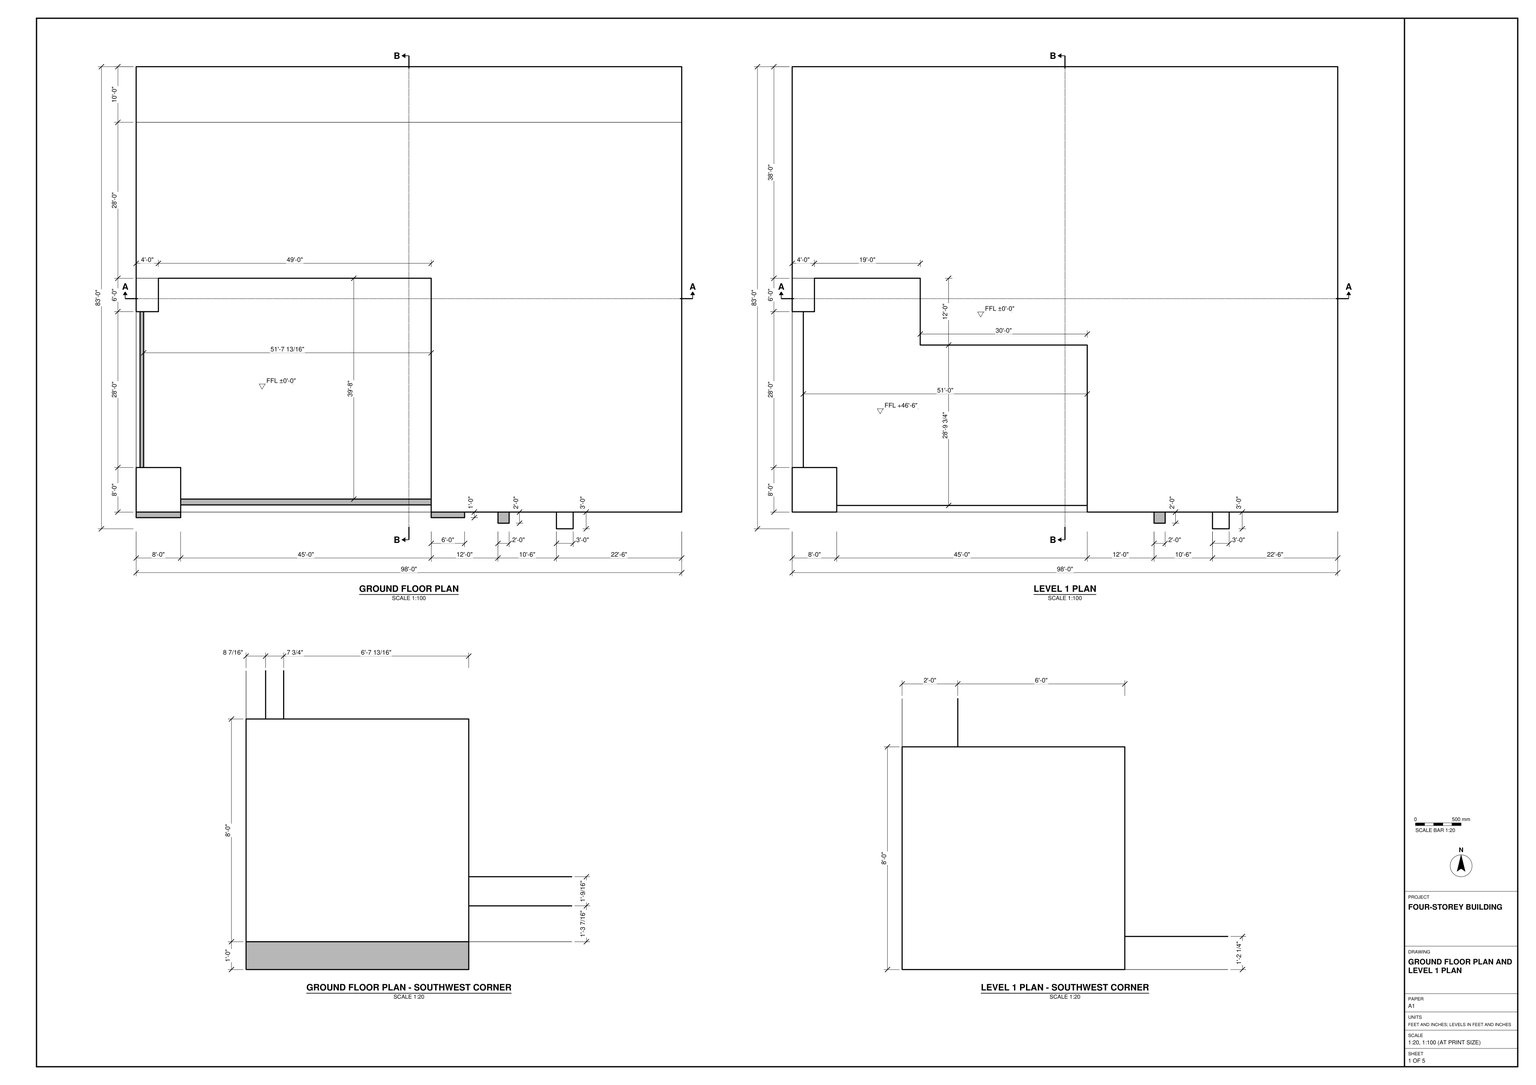
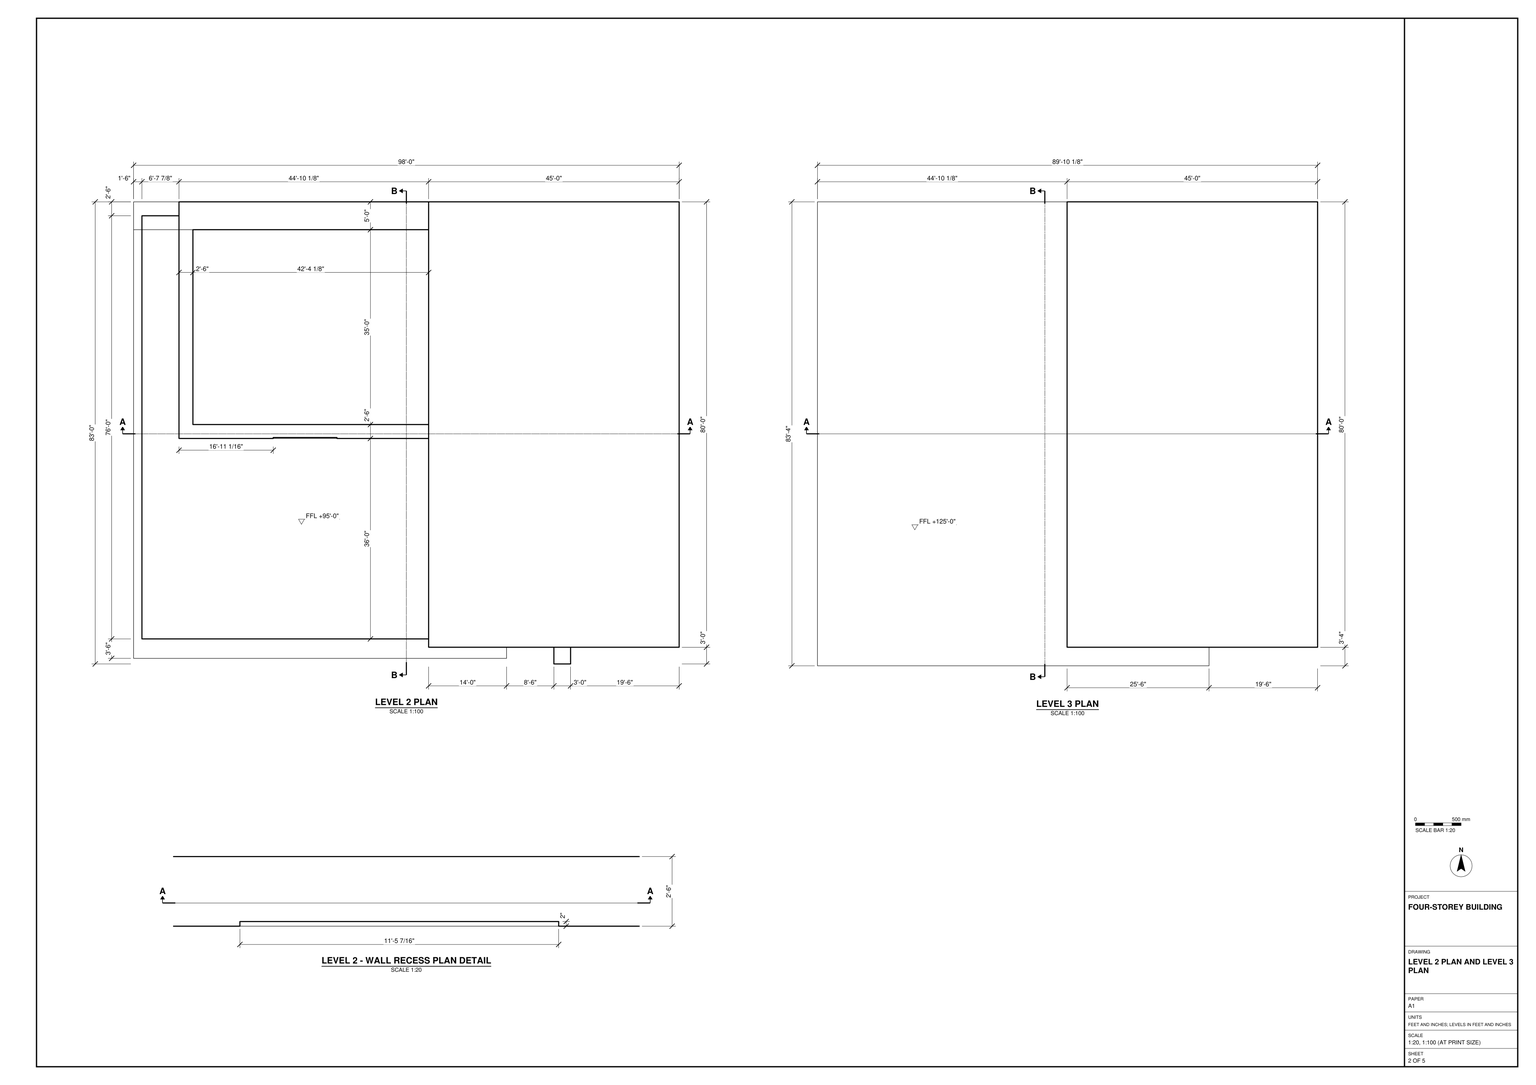
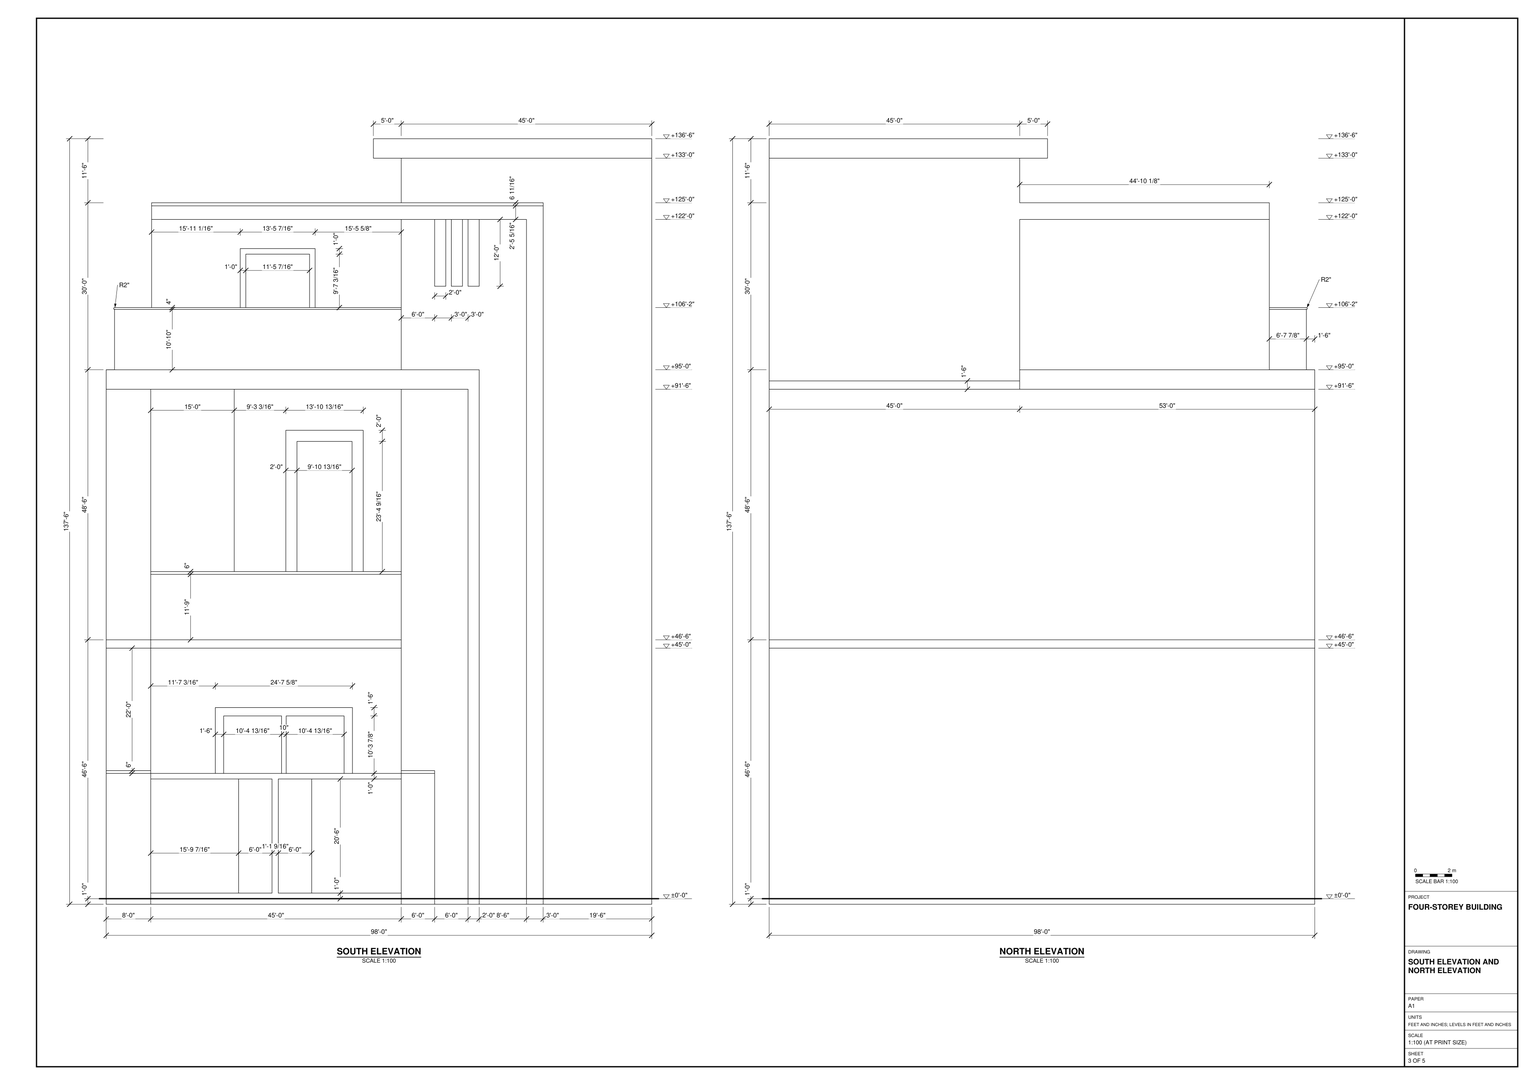
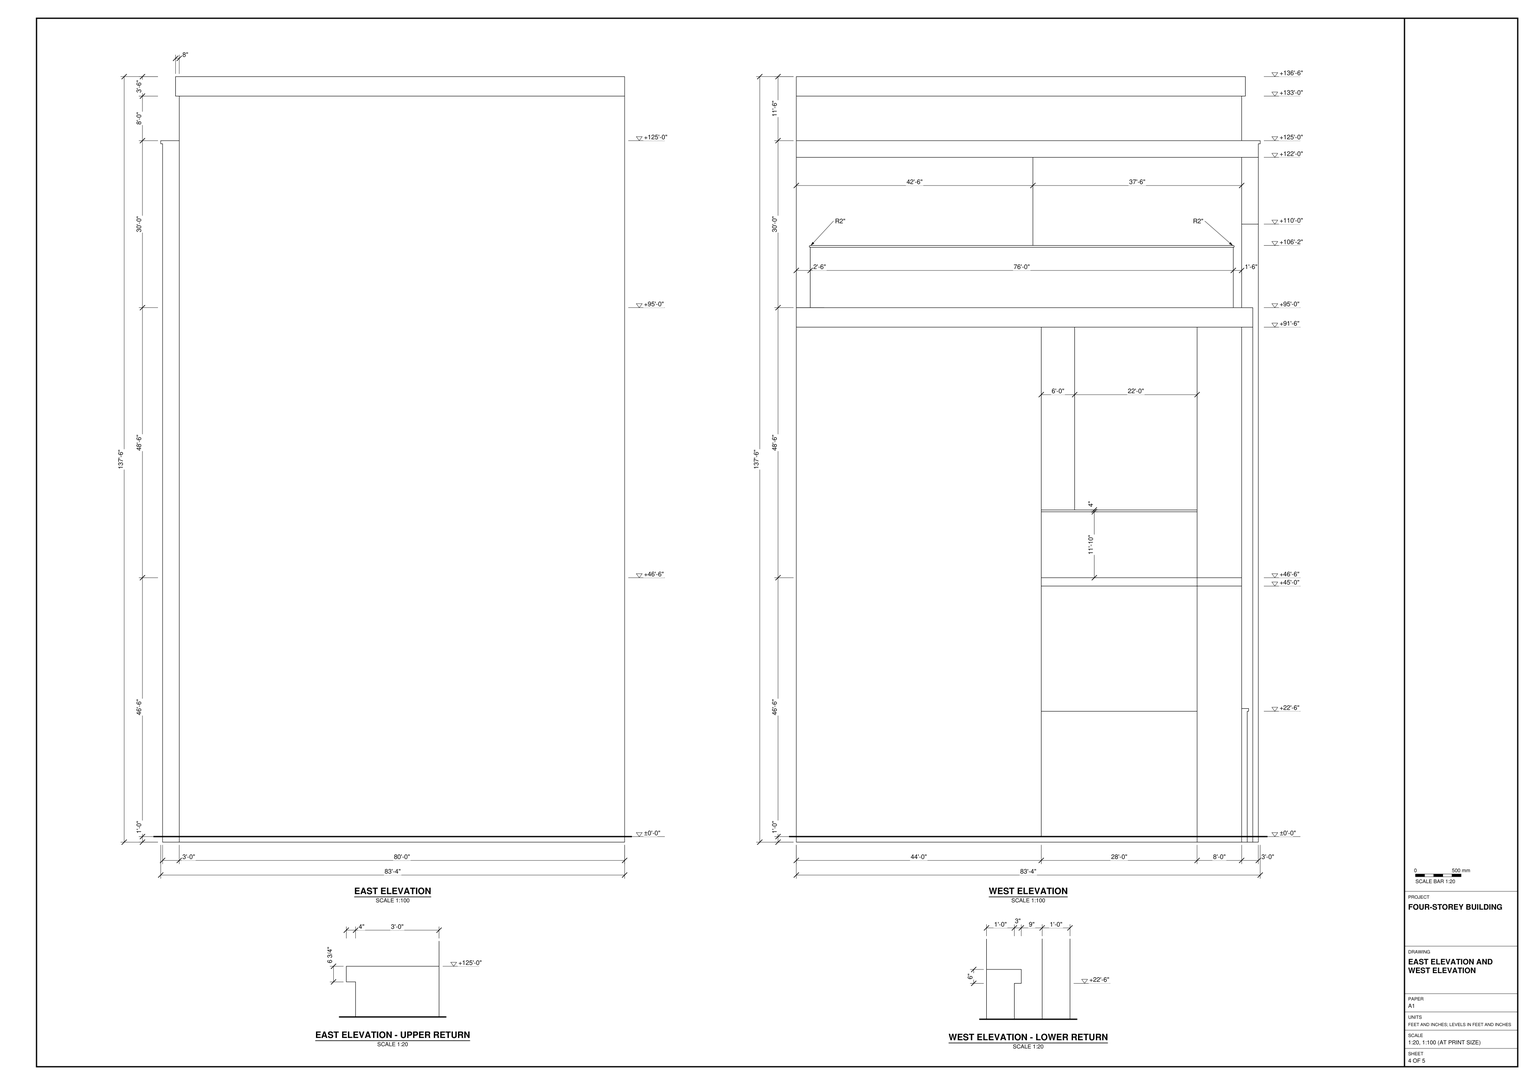
Build the four-storey building in SketchUp from task_files/diagram_01.pdf. Work in feet and inches. The overall dimensions are 98'-0" east to west, 83'-4" north to south and 137'-6" from the underside of the base to the top of the roof. Set the ground floor at ±0'-0" and the successive floor levels at +46'-6", +95'-0" and +125'-0".

Use the floor plans to locate the walls, slab edges and supports. Follow the enlarged southwest corner details: the adjoining edges meet the corner pier at different offsets on the ground floor and Level 1. Form the stepped bay on Level 1 and the shallow wall recess on Level 2. Use the wall and slab thicknesses shown rather than giving all elements a common thickness.

Match the south elevation’s framed openings, horizontal bands and vertical returns. Keep the highest volume on the east side and extend its flat roof cap westward as drawn. Group walls, slabs and roofs separately. Keep each furniture or joinery piece shown in its own group or component, and use components for repeated parts. Decor and loose items may be any suitable library components. Save one SketchUp model as output_files/four_storey_building_with_stepped_facades.skp.

# SketchUp Ruby script. Lengths in inches.
U = 1.inch
M = Sketchup.active_model
def pt(a) = Geom::Point3d.new(a.map { |v| v * U })
def face(e, loops, mat)
  f = e.add_face(loops[0].map { |a| pt(a) })
  loops[1..].each { |l| e.add_face(l.map { |a| pt(a) }).erase! }
  f.material = f.back_material = mat if mat
  f
end
# faces: each face lists its corners as indices into pts; further lists are holes
def faces(e, pts, list, mat = nil) = list.each { |f| face(e, (f[0].is_a?(Array) ? f : [f]).map { |l| l.map { |i| pts[i] } }, mat) }
# xy, xz, yz: faces in a plane at the given z, y or x. An outline is a flat list of corners, or four numbers for a rectangle; further outlines are holes
def ring(l) = l.size == 4 ? [[l[0], l[1]], [l[2], l[1]], [l[2], l[3]], [l[0], l[3]]] : l.each_slice(2).to_a
def flat(e, list, mat, &to3) = list.each { |f| face(e, (f[0].is_a?(Array) ? f : [f]).map { |l| ring(l).map { |u, v| to3.(u, v) } }, mat) }
def xy(e, z, list, mat = nil) = flat(e, list, mat) { |x, y| [x, y, z] }
def xz(e, y, list, mat = nil) = flat(e, list, mat) { |x, z| [x, y, z] }
def yz(e, x, list, mat = nil) = flat(e, list, mat) { |y, z| [x, y, z] }
def lines(e, pts, list) = list.each { |a, b| e.add_line(pt(pts[a]), pt(pts[b])) }
# prism: a flat outline (further loops are holes) pulled along v
def prism(e, loops, v, mat = nil)
  f = face(e, loops, mat); d = Geom::Vector3d.new(v.map { |x| x * U })
  f.pushpull(f.normal.samedirection?(d) ? d.length : -d.length)
end
def box(e, o, s, mat = nil) = prism(e, [[o, [o[0] + s[0], o[1], o[2]], [o[0] + s[0], o[1] + s[1], o[2]], [o[0], o[1] + s[1], o[2]]]], [0, 0, s[2]], mat)
def at(x, y, z, deg = 0) = Geom::Transformation.translation(pt([x, y, z])) * Geom::Transformation.rotation(ORIGIN, Z_AXIS, deg.degrees)
def axes(o, x, y, z) = Geom::Transformation.new([*x, 0, *y, 0, *z, 0, *pt(o).to_a, 1])
def part(name) = M.definitions.add(name)
# library, detail: a bought-in or finely detailed component or shape, given as its bounding box
def library(name, o, s) = part(name).tap { |d| box(d.entities, o, s) }
def detail(e, o, s) = box(e.add_group.entities, o, s)
def put(e, d, t, mat = nil) = e.add_instance(d, t).tap { |i| i.material = mat if mat }
def group(e, t, mat = nil) = e.add_group.tap { |g| g.transformation = t; g.material = mat if mat }.entities
root = M.entities
M.materials.add("[0009_Linen]").color = [250, 240, 230]
M.materials.add("[0051_Cornsilk]").color = [255, 248, 220]
M.materials.add("[0061_OliveDrab]").color = [53, 71, 17]
M.materials.add("[0061_OliveDrab]1").color = [71, 94, 23]
M.materials.add("[0118_Thistle]").color = [216, 191, 216]
M.materials.add("[0132_LightGray]").color = [169, 169, 169]
M.materials.add("[0135_DarkGray]").color = [81, 81, 81]
M.materials.add("[0136_Charcoal]").color = [17, 17, 17]
M.materials.add("[Carrera Marble]").color = [165, 165, 165]
M.materials.add("[Checker Plate]").color = [247, 247, 247]
M.materials.add("[Cladding Siding Tan]").color = [90, 119, 67]
M.materials.add("[Cladding Siding Tan]1").color = [127, 71, 26]
M.materials.add("[Stone Marble]").color = [143, 138, 136]
M.materials.add("[Translucent Glass Gray]").color = [128, 128, 128]
M.materials["[Translucent Glass Gray]"].alpha = 0.5
xy(root,0,[[906,4,942,40],[780,16,804,40],[0,28,96,40],[636,28,708,40],[0,40,1176,880],
  [0,880,1176,1000]])
xy(root,12,[[96,55.44,636,68.01],[8.43,136,16.2,472],[0,472,48,544]])
xy(root,12,[[96,40,636,55.44],[96,68.01,636,68.01,636,544,48,544,48,472,16.2,472,16.2,136,96,136],[0,136,8.43,472]],"[Stone Marble]")
xy(root,126.9,[[253.2,544,378.01,546],[388.01,544,512.83,546]])
xy(root,282,[[0,25,96,28],[636,25,708,28]])
xy(root,282,[[96,55.44,636,68.01],[8.43,136,16.2,472]],"[0009_Linen]")
xy(root,288,[[0,25,96,40],[636,25,708,40]],"[0061_OliveDrab]")
xy(root,405.9,[[253.2,544,378.01,546],[388.01,544,512.83,546]])
xy(root,552,[[220.83,139.21,217.72,139.57,214.81,140.72,212.29,142.58,210.34,145.03,209.09,147.9,208.63,151,208.98,154.12,210.13,157.03,212,159.55,214.45,161.5,217.32,162.75,220.42,163.21,223.53,162.85,226.45,161.7,228.96,159.84,230.91,157.39,232.16,154.52,232.625,151.42,232.27,148.3,231.12,145.39,229.26,142.87,226.8,140.92,223.93,139.67],[444.46,139.21,441.35,139.57,438.43,140.72,435.91,142.58,433.96,145.03,432.72,147.9,432.25,151,432.61,154.12,433.76,157.03,435.62,159.55,438.07,161.5,440.95,162.75,444.04,163.21,447.16,162.85,450.07,161.7,452.59,159.84,454.54,157.39,455.79,154.52,456.25,151.42,455.89,148.3,454.75,145.39,452.88,142.87,450.43,140.92,447.56,139.67],[198.83,349.52,195.72,349.88,192.81,351.03,190.29,352.89,188.34,355.34,187.09,358.22,186.63,361.32,186.98,364.43,188.13,367.34,190,369.86,192.45,371.81,195.32,373.06,198.42,373.52,201.53,373.17,204.45,372.02,206.96,370.15,208.91,367.7,210.16,364.83,210.625,361.73,210.27,358.62,209.12,355.7,207.26,353.18,204.8,351.24,201.93,349.99],[444.46,349.52,441.35,349.88,438.43,351.03,435.91,352.89,433.96,355.34,432.72,358.22,432.25,361.32,432.61,364.43,433.76,367.34,435.62,369.86,438.07,371.81,440.95,373.06,444.04,373.52,447.16,373.17,450.07,372.02,452.59,370.15,454.54,367.7,455.79,364.83,456.25,361.73,455.89,358.62,454.75,355.7,452.88,353.18,450.43,351.24,447.56,349.99]])
xy(root,552,[[[96,40,96,136,0,136,0,472,48,472,48,544,636,544,636,40],[220.83,139.21,223.93,139.67,226.8,140.92,229.26,142.87,231.12,145.39,232.27,148.3,232.625,151.42,232.16,154.52,230.91,157.39,228.96,159.84,226.45,161.7,223.53,162.85,220.42,163.21,217.32,162.75,214.45,161.5,212,159.55,210.13,157.03,208.98,154.12,208.63,151,209.09,147.9,210.34,145.03,212.29,142.58,214.81,140.72,217.72,139.57],[444.46,139.21,447.56,139.67,450.43,140.92,452.88,142.87,454.75,145.39,455.89,148.3,456.25,151.42,455.79,154.52,454.54,157.39,452.59,159.84,450.07,161.7,447.16,162.85,444.04,163.21,440.95,162.75,438.07,161.5,435.62,159.55,433.76,157.03,432.61,154.12,432.25,151,432.72,147.9,433.96,145.03,435.91,142.58,438.43,140.72,441.35,139.57],[444.46,349.52,447.56,349.99,450.43,351.24,452.88,353.18,454.75,355.7,455.89,358.62,456.25,361.73,455.79,364.83,454.54,367.7,452.59,370.15,450.07,372.02,447.16,373.17,444.04,373.52,440.95,373.06,438.07,371.81,435.62,369.86,433.76,367.34,432.61,364.43,432.25,361.32,432.72,358.22,433.96,355.34,435.91,352.89,438.43,351.03,441.35,349.88],[198.83,349.52,201.93,349.99,204.8,351.24,207.26,353.18,209.12,355.7,210.27,358.62,210.625,361.73,210.16,364.83,208.91,367.7,206.96,370.15,204.45,372.02,201.53,373.17,198.42,373.52,195.32,373.06,192.45,371.81,190,369.86,188.13,367.34,186.98,364.43,186.63,361.32,187.09,358.22,188.34,355.34,190.29,352.89,192.81,351.03,195.72,349.88]]],"[0118_Thistle]")
xy(root,570,[[0,40,96,136]])
xy(root,570,[[96,40,636,54.26],[0,136,24,472]],"[0051_Cornsilk]")
xy(root,570,[[96,54.26,636,54.26,636,400,276,400,276,544,48,544,48,472,24,472,24,136,96,136]],"[Carrera Marble]")
xy(root,657.21,[[411.19,400,530.01,402]])
xy(root,997.58,[[411.19,400,530.01,402]])
xy(root,1110,[[0,16,96,40],[215.45,103.5,212.32,103.56,209.31,104.42,206.62,106.03,204.44,108.28,202.92,111.02,202.16,114.0625,202.22,117.19,203.08,120.2,204.69,122.89,206.94,125.07,209.68,126.59,212.72,127.35,215.85,127.3,218.86,126.43,221.55,124.82,223.73,122.57,225.25,119.83,226.01,116.79,225.96,113.66,225.09,110.65,223.48,107.96,221.23,105.78,218.49,104.26],[467.01,103.5,463.88,103.56,460.87,104.42,458.18,106.03,456.01,108.28,454.49,111.02,453.73,114.0625,453.78,117.19,454.64,120.2,456.25,122.89,458.51,125.07,461.24,126.59,464.28,127.35,467.42,127.3,470.43,126.43,473.11,124.82,475.29,122.57,476.8125,119.83,477.57,116.79,477.52,113.66,476.66,110.65,475.04,107.96,472.79,105.78,470.05,104.26],[197.51,304.07,194.38,304.12,191.37,304.98,188.68,306.59,186.51,308.85,184.99,311.58,184.23,314.625,184.28,317.76,185.14,320.77,186.75,323.45,189.01,325.63,191.74,327.15,194.78,327.91,197.92,327.86,200.93,327,203.61,325.38,205.79,323.13,207.3125,320.39,208.07,317.35,208.02,314.22,207.16,311.21,205.54,308.52,203.29,306.35,200.55,304.83],[467.01,304.07,463.88,304.12,460.87,304.98,458.18,306.59,456.01,308.85,454.49,311.58,453.73,314.625,453.78,317.76,454.64,320.77,456.25,323.45,458.51,325.63,461.24,327.15,464.28,327.91,467.42,327.86,470.43,327,473.11,325.38,475.29,323.13,476.8125,320.39,477.57,317.35,477.52,314.22,476.66,311.21,475.04,308.52,472.79,306.35,470.05,304.83],
  [0,472,48,544]])
xy(root,1110,[[[96,16,96,136,0,136,0,472,48,472,48,544,276,544,276,400,636,400,636,40,780,40,780,16],[215.45,103.5,218.49,104.26,221.23,105.78,223.48,107.96,225.09,110.65,225.96,113.66,226.01,116.79,225.25,119.83,223.73,122.57,221.55,124.82,218.86,126.43,215.85,127.3,212.72,127.35,209.68,126.59,206.94,125.07,204.69,122.89,203.08,120.2,202.22,117.19,202.16,114.0625,202.92,111.02,204.44,108.28,206.62,106.03,209.31,104.42,212.32,103.56],[467.01,103.5,470.05,104.26,472.79,105.78,475.04,107.96,476.66,110.65,477.52,113.66,477.57,116.79,476.8125,119.83,475.29,122.57,473.11,124.82,470.43,126.43,467.42,127.3,464.28,127.35,461.24,126.59,458.51,125.07,456.25,122.89,454.64,120.2,453.78,117.19,453.73,114.0625,454.49,111.02,456.01,108.28,458.18,106.03,460.87,104.42,463.88,103.56],[467.01,304.07,470.05,304.83,472.79,306.35,475.04,308.52,476.66,311.21,477.52,314.22,477.57,317.35,476.8125,320.39,475.29,323.13,473.11,325.38,470.43,327,467.42,327.86,464.28,327.91,461.24,327.15,458.51,325.63,456.25,323.45,454.64,320.77,453.78,317.76,453.73,314.625,454.49,311.58,456.01,308.85,458.18,306.59,460.87,304.98,463.88,304.12],[197.51,304.07,200.55,304.83,203.29,306.35,205.54,308.52,207.16,311.21,208.02,314.22,208.07,317.35,207.3125,320.39,205.79,323.13,203.61,325.38,200.93,327,197.92,327.86,194.78,327.91,191.74,327.15,189.01,325.63,186.75,323.45,185.14,320.77,184.28,317.76,184.23,314.625,184.99,311.58,186.51,308.85,188.68,306.59,191.37,304.98,194.38,304.12]]],"[0118_Thistle]")
xy(root,1152,[[97.875,490,97.875,940,127.875,940,127.875,520,636,520,636,490],[127.875,520,636,940],[0,940,97.875,1000],[97.875,940,636,1000]])
xy(root,1152,[[0,16,804,16,804,40,636,40,636,58,18,58,18,940,0,940]],"[0051_Cornsilk]")
xy(root,1152,[[18,58,636,58,636,490,97.875,490,97.875,940,18,940]],"[Carrera Marble]")
xy(root,1152.1,[[0,940,97.875,1000]],"[0051_Cornsilk]")
xy(root,1164,[[300.93,490,438.37,492]])
xy(root,1332,[[708,4,732,40],[744,4,768,40],[780,4,804,40]],"[0135_DarkGray]")
xy(root,1401.21,[[300.93,490,438.37,492]])
xy(root,1476,[[708,4,732,40],[744,4,768,40],[780,4,804,40],[236.73,103.47,233.59,103.5,230.58,104.34,227.875,105.93,225.68,108.16,224.14,110.89,223.35,113.92,223.38,117.05,224.22,120.07,225.8,122.77,228.04,124.97,230.76,126.51,233.8,127.29,236.93,127.27,239.95,126.43,242.65,124.84,244.84,122.61,246.39,119.88,247.17,116.85,247.15,113.72,246.31,110.7,244.72,108,242.49,105.8,239.76,104.26],[459.04,103.47,455.91,103.5,452.89,104.34,450.1875,105.93,447.99,108.16,446.45,110.89,445.66,113.92,445.69,117.05,446.53,120.07,448.12,122.77,450.35,124.97,453.08,126.51,456.11,127.29,459.24,127.27,462.26,126.43,464.96,124.84,467.16,122.61,468.7,119.88,469.48,116.85,469.46,113.72,468.62,110.7,467.03,108,464.8,105.8,462.07,104.26],
  [216.91,321.22,213.78,321.25,210.76,322.09,208.0625,323.68,205.87,325.91,204.32,328.64,203.54,331.67,203.57,334.8,204.4,337.82,205.99,340.52,208.23,342.72,210.95,344.26,213.98,345.04,217.12,345.02,220.14,344.18,222.84,342.59,225.03,340.36,226.57,337.63,227.36,334.6,227.33,331.47,226.5,328.45,224.91,325.75,222.67,323.55,219.95,322.01],[459.04,321.22,455.91,321.25,452.89,322.09,450.1875,323.68,447.99,325.91,446.45,328.64,445.66,331.67,445.69,334.8,446.53,337.82,448.12,340.52,450.35,342.72,453.08,344.26,456.11,345.04,459.24,345.02,462.26,344.18,464.96,342.59,467.16,340.36,468.7,337.63,469.48,334.6,469.46,331.47,468.62,328.45,467.03,325.75,464.8,323.55,462.07,322.01],[97.875,490,636,490,636,520,127.875,520,127.875,940,97.875,940],[127.875,520,636,940],[97.875,940,636,1000]])
xy(root,1476,[[804,4,906,40]],"[0009_Linen]")
xy(root,1476,[[[97.875,4,97.875,490,636,490,636,40,708,40,708,4],[459.04,103.47,462.07,104.26,464.8,105.8,467.03,108,468.62,110.7,469.46,113.72,469.48,116.85,468.7,119.88,467.16,122.61,464.96,124.84,462.26,126.43,459.24,127.27,456.11,127.29,453.08,126.51,450.35,124.97,448.12,122.77,446.53,120.07,445.69,117.05,445.66,113.92,446.45,110.89,447.99,108.16,450.1875,105.93,452.89,104.34,455.91,103.5],[459.04,321.22,462.07,322.01,464.8,323.55,467.03,325.75,468.62,328.45,469.46,331.47,469.48,334.6,468.7,337.63,467.16,340.36,464.96,342.59,462.26,344.18,459.24,345.02,456.11,345.04,453.08,344.26,450.35,342.72,448.12,340.52,446.53,337.82,445.69,334.8,445.66,331.67,446.45,328.64,447.99,325.91,450.1875,323.68,452.89,322.09,455.91,321.25],[216.91,321.22,219.95,322.01,222.67,323.55,224.91,325.75,226.5,328.45,227.33,331.47,227.36,334.6,226.57,337.63,225.03,340.36,222.84,342.59,220.14,344.18,217.12,345.02,213.98,345.04,210.95,344.26,208.23,342.72,205.99,340.52,204.4,337.82,203.57,334.8,203.54,331.67,204.32,328.64,205.87,325.91,208.0625,323.68,210.76,322.09,213.78,321.25],[236.73,103.47,239.76,104.26,242.49,105.8,244.72,108,246.31,110.7,247.15,113.72,247.17,116.85,246.39,119.88,244.84,122.61,242.65,124.84,239.95,126.43,236.93,127.27,233.8,127.29,230.76,126.51,228.04,124.97,225.8,122.77,224.22,120.07,223.38,117.05,223.35,113.92,224.14,110.89,225.68,108.16,227.875,105.93,230.58,104.34,233.59,103.5]]],"[0118_Thistle]")
xy(root,1476,[[732,4,744,40],[768,4,780,40]],"[0132_LightGray]")
xy(root,1505.29,[[97.875,0,942,4]])
xy(root,1512,[[97.875,0,942,0,942,40,636,40,636,1000,97.875,1000]],"[0051_Cornsilk]")
xy(root,1608,[[576,32,576,1000,636,1000,636,40,1176,40,1176,32],[636,40,1176,1000]])
xy(root,1650,[[576,32,1176,1000]],"[0051_Cornsilk]")
xz(root,0,[[97.875,1505.29,942,1512]],"[0051_Cornsilk]")
xz(root,4,[[906,0,942,0,942,1505.29,97.875,1505.29,97.875,1476,906,1476]],"[0051_Cornsilk]")
xz(root,4,[[708,1332,732,1476],[744,1332,768,1476],[780,1332,804,1476]],"[0135_DarkGray]")
xz(root,16,[[780,0,804,0,804,1152,0,1152,0,1110,780,1110]],"[0051_Cornsilk]")
xz(root,25,[[0,282,96,288],[636,282,708,288]],"[0051_Cornsilk]")
xz(root,28,[[0,0,96,282],[636,0,708,282]],"[0061_OliveDrab]")
xz(root,32,[[576,1608,1176,1650]],"[0051_Cornsilk]")
xz(root,40,[[0,0,96,12],[636,0,708,282],[780,0,804,1110],[906,0,942,12],[0,12,96,282],
  [906,12,906,1476,636,1476,636,1512,942,1512,942,12],[0,282,96,288],[636,282,708,288],[636,1110,804,1152],[708,1332,732,1476],
  [744,1332,768,1476],[780,1332,804,1476]])
xz(root,40,[[0,552,96,570],[96,552,636,570]],"[0051_Cornsilk]")
xz(root,40,[[0,288,96,552],[0,570,96,1110]],"[0061_OliveDrab]")
xz(root,40,[[708,0,780,0,780,1110,636,1110,636,288,708,288],[804,0,906,0,906,1476,804,1476,804,1332,780,1332,780,1476,768,1476,768,1332,744,1332,744,1476,732,1476,732,1332,708,1332,708,1476,636,1476,636,1152,804,1152],[942,0,1176,0,1176,1608,636,1608,636,1512,942,1512]],"[Cladding Siding Tan]")
xz(root,40,[[96,0,636,12]],"[Stone Marble]")
xz(root,54.26,[[96,711,636,714]])
xz(root,54.26,[[96,570,636,711]],"[Translucent Glass Gray]")
xz(root,55.44,[[96,12,285.46,24],[285.46,12,357.46,24],[357.46,12,371,24],[371,12,443,24],[443,12,636,24],
  [357.46,24,371,24,371,270,636,270,636,282,96,282,96,270,357.46,270]],"[0061_OliveDrab]1")
xz(root,55.44,[[285.46,24,357.46,270],[371,24,443,270]],"[Checker Plate]")
xz(root,55.44,[[96,24,285.46,270],[443,24,636,270]],"[Cladding Siding Tan]1")
xz(root,58,[[18,1282,636,1284]])
xz(root,58,[[18,1152,636,1282]],"[Translucent Glass Gray]")
xz(root,68.01,[[96,12,636,282]])
xz(root,136,[[0,12,0,552,96,552,96,12,16.2,12,16.2,282,8.43,282,8.43,12],[8.43,12,16.2,282]])
xz(root,136,[[[0,570,96,1110],[24.23,712.01,24.73,712.14,25.1875,712.39,25.5625,712.75,25.83,713.2,25.98,713.7,25.99,714.23,25.86,714.73,25.61,715.1875,25.25,715.5625,24.8,715.83,24.3,715.98,23.77,715.99,23.27,715.86,22.8125,715.61,22.4375,715.25,22.17,714.8,22.02,714.3,22.01,713.77,22.14,713.27,22.39,712.8125,22.75,712.4375,23.2,712.17,23.7,712.02,24,712.02]]],"[0061_OliveDrab]")
xz(root,400,[[[387.19,633.21,554.01,1021.58],[411.19,657.21,530.01,997.58]]],"[0136_Charcoal]")
xz(root,400,[[[276,570,636,1110],[387.19,633.21,554.01,1021.58]]],"[Cladding Siding Tan]")
xz(root,402,[[411.19,657.21,530.01,997.58]],"[Translucent Glass Gray]")
xz(root,472,[[8.43,12,16.2,282],[24.23,712.01,24,712.02,23.7,712.02,23.2,712.17,22.75,712.4375,22.39,712.8125,22.14,713.27,22.01,713.77,22.02,714.3,22.17,714.8,22.4375,715.25,22.8125,715.61,23.27,715.86,23.77,715.99,24.3,715.98,24.8,715.83,25.25,715.5625,25.61,715.1875,25.86,714.73,25.99,714.23,25.98,713.7,25.83,713.2,25.5625,712.75,25.1875,712.39,24.73,712.14]])
xz(root,472,[[0,12,8.43,12,8.43,282,16.2,282,16.2,12,48,12,48,552,0,552],[[0,570,48,1110],[24.23,712.01,24,712.02,23.7,712.02,23.2,712.17,22.75,712.4375,22.39,712.8125,22.14,713.27,22.01,713.77,22.02,714.3,22.17,714.8,22.4375,715.25,22.8125,715.61,23.27,715.86,23.77,715.99,24.3,715.98,24.8,715.83,25.25,715.5625,25.61,715.1875,25.86,714.73,25.99,714.23,25.98,713.7,25.83,713.2,25.5625,712.75,25.1875,712.39,24.73,712.14]]],"[0061_OliveDrab]")
xz(root,490,[[[288.93,1152,450.37,1413.21],[300.93,1164,438.37,1401.21]]],"[0136_Charcoal]")
xz(root,490,[[97.875,1152,288.93,1152,288.93,1413.21,450.37,1413.21,450.37,1152,636,1152,636,1476,97.875,1476]],"[Cladding Siding Tan]")
xz(root,492,[[300.93,1164,438.37,1401.21]],"[Translucent Glass Gray]")
xz(root,520,[[127.875,1152,636,1476]])
xz(root,544,[[[235.2,108.9,530.83,423.9],[253.2,126.9,378.01,405.9],[388.01,126.9,512.83,405.9]]],"[0136_Charcoal]")
xz(root,544,[[[48,12,636,552],[235.2,108.9,530.83,423.9]],[48,570,276,1110]],"[Cladding Siding Tan]")
xz(root,546,[[253.2,126.9,378.01,405.9],[388.01,126.9,512.83,405.9]],"[Translucent Glass Gray]")
xz(root,940,[[0,1152,97.875,1152.1],[127.875,1152,636,1476]])
xz(root,970,[[18,1282,97.875,1284]])
xz(root,970,[[18,1152,97.875,1152.1,97.875,1282,18,1282]],"[Translucent Glass Gray]")
xz(root,1000,[[0,0,1176,12],[0,12,1176,552],[0,552,1176,570],[0,570,1176,1110],[0,1110,636,1152],
  [636,1110,1176,1128],[636,1128,636,1476,97.875,1476,97.875,1512,636,1512,636,1608,1176,1608,1176,1128],[0,1152,97.875,1152.1],[97.875,1152,636,1476],[576,1608,1176,1650]])
yz(root,0,[[940,1152,1000,1152.1]])
yz(root,0,[[472,12,1000,1110]],"[0009_Linen]")
yz(root,0,[[40,552,136,570],[136,552,472,570],[16,1110,1000,1152]],"[0051_Cornsilk]")
yz(root,0,[[28,0,28,282,25,282,25,288,40,288,40,0],[40,0,136,552],[40,570,136,1110]],"[0061_OliveDrab]")
yz(root,0,[[136,0,1000,12]],"[Stone Marble]")
yz(root,8.43,[[136,12,472,282]],"[0061_OliveDrab]")
yz(root,16.2,[[136,12,472,282]],"[0061_OliveDrab]")
yz(root,18,[[58,1282,970,1284]])
yz(root,18,[[58,1152,970,1282]],"[Translucent Glass Gray]")
yz(root,24,[[136,570,472,714]],"[Translucent Glass Gray]")
yz(root,48,[[472,12,544,552],[472,570,544,1110]],"[0061_OliveDrab]")
yz(root,96,[[55.44,12,68.01,282]])
yz(root,96,[[28,0,40,0,40,288,25,288,25,282,28,282],[40,12,55.44,12,55.44,282,68.01,282,68.01,12,136,12,136,552,40,552],[[40,570,136,1110],[54.26,711,53.95,711.02,53.64,711.07,53.34,711.15,53.04,711.26,52.76,711.4,52.5,711.57,52.26,711.77,52.03,711.99,51.84,712.24,51.66,712.5,51.52,712.78,51.41,713.07,51.33,713.375,51.28,713.6875,51.26,714,51.28,714.3125,51.33,714.625,51.41,714.93,51.52,715.22,51.66,715.5,51.84,715.76,52.03,716.01,52.26,716.23,52.5,716.43,52.76,716.6,53.04,716.74,53.34,716.85,53.64,716.93,53.95,716.98,54.26,717,54.58,716.98,54.89,716.93,55.19,716.85,55.48,716.74,55.76,716.6,56.03,716.43,56.27,716.23,56.49,716.01,56.69,715.76,56.86,715.5,57,715.22,57.12,714.93,57.2,714.625,57.25,714.3125,57.26,714,57.25,713.6875,57.2,713.375,57.12,713.07,57,712.78,56.86,712.5,56.69,712.24,56.49,711.99,56.27,711.77,56.03,711.57,55.76,711.4,55.48,711.26,55.19,711.15,54.89,711.07,54.58,711.02]]],"[0061_OliveDrab]")
yz(root,97.875,[[940,1152,1000,1152.1],[970,1282,970.21,1282.01,970.42,1282.04,970.62,1282.1,970.8125,1282.17,971,1282.27,971.18,1282.38,971.34,1282.51,971.49,1282.66,971.62,1282.82,971.73,1283,971.83,1283.1875,971.9,1283.38,971.96,1283.58,971.99,1283.79,972,1284,971.99,1284.21,971.96,1284.42,971.9,1284.62,971.83,1284.8125,971.73,1285,971.62,1285.18,971.49,1285.34,971.34,1285.49,971.18,1285.62,971,1285.73,970.8125,1285.83,970.62,1285.9,970.42,1285.96,970.21,1285.99,970,1286,969.79,1285.99,969.58,1285.96,969.38,1285.9,969.1875,1285.83,969,1285.73,968.82,1285.62,968.66,1285.49,968.51,1285.34,968.38,1285.18,968.27,1285,968.17,1284.8125,968.1,1284.62,968.04,1284.42,968.01,1284.21,968,1284,968.01,1283.79,968.04,1283.58,968.1,1283.38,968.17,1283.1875,968.27,1283,968.38,1282.82,968.51,1282.66,968.66,1282.51,968.82,1282.38,969,1282.27,969.1875,1282.17,969.38,1282.1,969.58,1282.04,969.79,1282.01]])
yz(root,97.875,[[4,1476,4,1505.29,0,1505.29,0,1512,1000,1512,1000,1476]],"[0009_Linen]")
yz(root,97.875,[[[490,1152,490,1476,1000,1476,1000,1152.1,940,1152.1,940,1152],[970,1282,970.21,1282.01,970.42,1282.04,970.62,1282.1,970.8125,1282.17,971,1282.27,971.18,1282.38,971.34,1282.51,971.49,1282.66,971.62,1282.82,971.73,1283,971.83,1283.1875,971.9,1283.38,971.96,1283.58,971.99,1283.79,972,1284,971.99,1284.21,971.96,1284.42,971.9,1284.62,971.83,1284.8125,971.73,1285,971.62,1285.18,971.49,1285.34,971.34,1285.49,971.18,1285.62,971,1285.73,970.8125,1285.83,970.62,1285.9,970.42,1285.96,970.21,1285.99,970,1286,969.79,1285.99,969.58,1285.96,969.38,1285.9,969.1875,1285.83,969,1285.73,968.82,1285.62,968.66,1285.49,968.51,1285.34,968.38,1285.18,968.27,1285,968.17,1284.8125,968.1,1284.62,968.04,1284.42,968.01,1284.21,968,1284,968.01,1283.79,968.04,1283.58,968.1,1283.38,968.17,1283.1875,968.27,1283,968.38,1282.82,968.51,1282.66,968.66,1282.51,968.82,1282.38,969,1282.27,969.1875,1282.17,969.38,1282.1,969.58,1282.04,969.79,1282.01]]],"[Cladding Siding Tan]")
yz(root,127.875,[[520,1152,940,1476]])
yz(root,253.2,[[544,126.9,546,405.9]])
yz(root,276,[[400,570,544,1110]],"[Cladding Siding Tan]")
yz(root,300.93,[[490,1164,492,1401.21]])
yz(root,378.01,[[544,126.9,546,405.9]])
yz(root,388.01,[[544,126.9,546,405.9]])
yz(root,411.19,[[400,657.21,402,997.58]])
yz(root,438.37,[[490,1164,492,1401.21]])
yz(root,512.83,[[544,126.9,546,405.9]])
yz(root,530.01,[[400,657.21,402,997.58]])
yz(root,576,[[32,1608,1000,1650]],"[0009_Linen]")
yz(root,636,[[55.44,12,68.01,282],[54.26,711,54.58,711.02,54.89,711.07,55.19,711.15,55.48,711.26,55.76,711.4,56.03,711.57,56.27,711.77,56.49,711.99,56.69,712.24,56.86,712.5,57,712.78,57.12,713.07,57.2,713.375,57.25,713.6875,57.26,714,57.25,714.3125,57.2,714.625,57.12,714.93,57,715.22,56.86,715.5,56.69,715.76,56.49,716.01,56.27,716.23,56.03,716.43,55.76,716.6,55.48,716.74,55.19,716.85,54.89,716.93,54.58,716.98,54.26,717,53.95,716.98,53.64,716.93,53.34,716.85,53.04,716.74,52.76,716.6,52.5,716.43,52.26,716.23,52.03,716.01,51.84,715.76,51.66,715.5,51.52,715.22,51.41,714.93,51.33,714.625,51.28,714.3125,51.26,714,51.28,713.6875,51.33,713.375,51.41,713.07,51.52,712.78,51.66,712.5,51.84,712.24,52.03,711.99,52.26,711.77,52.5,711.57,52.76,711.4,53.04,711.26,53.34,711.15,53.64,711.07,53.95,711.02],[490,1152,520,1476],[520,1152,940,1476],[940,1152,1000,1308],
  [940,1308,1000,1368],[940,1368,1000,1476]])
yz(root,636,[[28,0,28,282,25,282,25,288,40,288,40,0]],"[0061_OliveDrab]")
yz(root,636,[[40,12,40,552,544,552,544,12,68.01,12,68.01,282,55.44,282,55.44,12],[[40,570,400,1110],[54.26,711,54.58,711.02,54.89,711.07,55.19,711.15,55.48,711.26,55.76,711.4,56.03,711.57,56.27,711.77,56.49,711.99,56.69,712.24,56.86,712.5,57,712.78,57.12,713.07,57.2,713.375,57.25,713.6875,57.26,714,57.25,714.3125,57.2,714.625,57.12,714.93,57,715.22,56.86,715.5,56.69,715.76,56.49,716.01,56.27,716.23,56.03,716.43,55.76,716.6,55.48,716.74,55.19,716.85,54.89,716.93,54.58,716.98,54.26,717,53.95,716.98,53.64,716.93,53.34,716.85,53.04,716.74,52.76,716.6,52.5,716.43,52.26,716.23,52.03,716.01,51.84,715.76,51.66,715.5,51.52,715.22,51.41,714.93,51.33,714.625,51.28,714.3125,51.26,714,51.28,713.6875,51.33,713.375,51.41,713.07,51.52,712.78,51.66,712.5,51.84,712.24,52.03,711.99,52.26,711.77,52.5,711.57,52.76,711.4,53.04,711.26,53.34,711.15,53.64,711.07,53.95,711.02]],[[40,1152,490,1476],[58,1282,58.21,1282.01,58.42,1282.04,58.62,1282.1,58.8125,1282.17,59,1282.27,59.18,1282.38,59.34,1282.51,59.49,1282.66,59.62,1282.82,59.73,1283,59.83,1283.1875,59.9,1283.38,59.96,1283.58,59.99,1283.79,60,1284,59.99,1284.21,59.96,1284.42,59.9,1284.62,59.83,1284.8125,59.73,1285,59.62,1285.18,59.49,1285.34,59.34,1285.49,59.18,1285.62,59,1285.73,58.8125,1285.83,58.62,1285.9,58.42,1285.96,58.21,1285.99,58,1286,57.79,1285.99,57.58,1285.96,57.38,1285.9,57.1875,1285.83,57,1285.73,56.82,1285.62,56.66,1285.49,56.51,1285.34,56.38,1285.18,56.27,1285,56.17,1284.8125,56.1,1284.62,56.04,1284.42,56.01,1284.21,56,1284,56.01,1283.79,56.04,1283.58,56.1,1283.38,56.17,1283.1875,56.27,1283,56.38,1282.82,56.51,1282.66,56.66,1282.51,56.82,1282.38,57,1282.27,57.1875,1282.17,57.38,1282.1,57.58,1282.04,57.79,1282.01]],[40,1512,1000,1608]],"[Cladding Siding Tan]")
yz(root,708,[[28,0,40,0,40,288,25,288,25,282,28,282]],"[0061_OliveDrab]")
yz(root,708,[[4,1332,40,1476]],"[0135_DarkGray]")
yz(root,732,[[4,1332,40,1476]],"[0135_DarkGray]")
yz(root,744,[[4,1332,40,1476]],"[0135_DarkGray]")
yz(root,768,[[4,1332,40,1476]],"[0135_DarkGray]")
yz(root,780,[[16,0,40,1110]],"[0051_Cornsilk]")
yz(root,780,[[4,1332,40,1476]],"[0135_DarkGray]")
yz(root,804,[[16,0,40,1152]],"[0051_Cornsilk]")
yz(root,804,[[4,1332,40,1476]],"[0135_DarkGray]")
yz(root,906,[[4,0,40,1476]],"[0051_Cornsilk]")
yz(root,942,[[4,0,40,0,40,1512,0,1512,0,1505.29,4,1505.29]],"[0051_Cornsilk]")
yz(root,1176,[[40,0,1000,1608],[32,1608,1000,1650]],"[0009_Linen]")
p = [[636,53.95,711.02],[636,53.64,711.07],[96,53.64,711.07],[96,53.95,711.02],[636,54.26,711],[96,54.26,711],
  [636,54.58,711.02],[96,54.58,711.02],[636,54.89,711.07],[96,54.89,711.07],[636,53.34,711.15],[636,53.04,711.26],
  [96,53.04,711.26],[96,53.34,711.15],[636,55.19,711.15],[96,55.19,711.15],[636,55.48,711.26],[96,55.48,711.26],
  [636,52.76,711.4],[96,52.76,711.4],[636,55.76,711.4],[96,55.76,711.4],[636,52.5,711.57],[96,52.5,711.57],
  [636,56.03,711.57],[96,56.03,711.57],[636,52.26,711.77],[96,52.26,711.77],[636,56.27,711.77],[96,56.27,711.77],
  [636,52.03,711.99],[96,52.03,711.99],[636,56.49,711.99],[96,56.49,711.99],[636,51.84,712.24],[96,51.84,712.24],
  [636,56.69,712.24],[96,56.69,712.24],[23.2,472,712.17],[23.7,472,712.02],[23.7,136,712.02],[23.2,136,712.17],
  [24,472,712.02],[24.23,472,712.01],[24.23,136,712.01],[24,136,712.02],[24.73,472,712.14],[24.73,136,712.14],
  [25.1875,472,712.39],[25.1875,136,712.39],[636,51.66,712.5],[96,51.66,712.5],[636,56.86,712.5],[96,56.86,712.5],
  [22.75,472,712.4375],[22.75,136,712.4375],[22.39,472,712.8125],[22.39,136,712.8125],[25.5625,472,712.75],[25.5625,136,712.75],
  [636,51.52,712.78],[96,51.52,712.78],[636,57,712.78],[96,57,712.78],[636,51.41,713.07],[96,51.41,713.07],
  [636,57.12,713.07],[96,57.12,713.07],[22.14,472,713.27],[22.14,136,713.27],[25.83,472,713.2],[25.83,136,713.2],
  [636,51.33,713.375],[96,51.33,713.375],[636,57.2,713.375],[96,57.2,713.375],[25.98,472,713.7],[25.98,136,713.7],
  [22.01,472,713.77],[22.01,136,713.77],[636,51.28,713.6875],[96,51.28,713.6875],[636,57.25,713.6875],[96,57.25,713.6875],
  [636,51.26,714],[96,51.26,714],[636,57.26,714],[96,57.26,714],[25.99,472,714.23],[25.99,136,714.23],
  [22.02,472,714.3],[22.02,136,714.3],[636,51.28,714.3125],[96,51.28,714.3125],[636,57.25,714.3125],[96,57.25,714.3125],
  [25.86,472,714.73],[25.86,136,714.73],[636,51.33,714.625],[96,51.33,714.625],[636,57.2,714.625],[96,57.2,714.625],
  [22.17,472,714.8],[22.17,136,714.8],[636,51.41,714.93],[96,51.41,714.93],[636,57.12,714.93],[96,57.12,714.93],
  [25.61,472,715.1875],[25.61,136,715.1875],[22.4375,472,715.25],[22.4375,136,715.25],[636,51.52,715.22],[96,51.52,715.22],
  [636,57,715.22],[96,57,715.22],[636,51.66,715.5],[96,51.66,715.5],[636,56.86,715.5],[96,56.86,715.5],
  [22.8125,472,715.61],[22.8125,136,715.61],[25.25,472,715.5625],[25.25,136,715.5625],[636,51.84,715.76],[96,51.84,715.76],
  [636,56.69,715.76],[96,56.69,715.76],[23.27,472,715.86],[23.27,136,715.86],[24.8,472,715.83],[24.8,136,715.83],
  [636,52.03,716.01],[96,52.03,716.01],[636,56.49,716.01],[96,56.49,716.01],[24.3,472,715.98],[24.3,136,715.98],
  [23.77,472,715.99],[23.77,136,715.99],[636,52.26,716.23],[96,52.26,716.23],[636,56.27,716.23],[96,56.27,716.23],
  [636,52.5,716.43],[96,52.5,716.43],[636,56.03,716.43],[96,56.03,716.43],[636,52.76,716.6],[96,52.76,716.6],
  [636,55.76,716.6],[96,55.76,716.6],[636,53.04,716.74],[96,53.04,716.74],[636,55.48,716.74],[96,55.48,716.74],
  [636,53.34,716.85],[96,53.34,716.85],[636,55.19,716.85],[96,55.19,716.85],[636,53.64,716.93],[96,53.64,716.93],
  [636,53.95,716.98],[96,53.95,716.98],[636,54.58,716.98],[636,54.89,716.93],[96,54.89,716.93],[96,54.58,716.98],
  [636,54.26,717],[96,54.26,717],[17.38,970.62,1282.1],[17.58,970.42,1282.04],[17.58,57.58,1282.04],[17.38,57.38,1282.1],
  [636,57.58,1282.04],[636,57.38,1282.1],[17.79,970.21,1282.01],[17.79,57.79,1282.01],[636,57.79,1282.01],[18,970,1282],
  [18,58,1282],[636,58,1282],[18.21,969.79,1282.01],[18.21,58.21,1282.01],[636,58.21,1282.01],[18.42,969.58,1282.04],
  [18.42,58.42,1282.04],[636,58.42,1282.04],[18.62,969.38,1282.1],[18.62,58.62,1282.1],[636,58.62,1282.1],[97.875,969.58,1282.04],
  [97.875,969.38,1282.1],[97.875,969.79,1282.01],[97.875,970,1282],[97.875,970.21,1282.01],[97.875,970.42,1282.04],[97.875,970.62,1282.1],
  [17.1875,970.8125,1282.17],[17.1875,57.1875,1282.17],[636,57.1875,1282.17],[18.8125,969.1875,1282.17],[18.8125,58.8125,1282.17],[636,58.8125,1282.17],
  [97.875,969.1875,1282.17],[97.875,970.8125,1282.17],[17,971,1282.27],[17,57,1282.27],[636,57,1282.27],[19,969,1282.27],
  [19,59,1282.27],[636,59,1282.27],[97.875,969,1282.27],[97.875,971,1282.27],[16.82,971.18,1282.38],[16.82,56.82,1282.38],
  [636,56.82,1282.38],[19.18,968.82,1282.38],[19.18,59.18,1282.38],[636,59.18,1282.38],[97.875,968.82,1282.38],[97.875,971.18,1282.38],
  [16.66,971.34,1282.51],[16.66,56.66,1282.51],[636,56.66,1282.51],[19.34,968.66,1282.51],[19.34,59.34,1282.51],[636,59.34,1282.51],
  [97.875,968.66,1282.51],[97.875,971.34,1282.51],[16.51,971.49,1282.66],[16.51,56.51,1282.66],[636,56.51,1282.66],[19.49,968.51,1282.66],
  [19.49,59.49,1282.66],[636,59.49,1282.66],[97.875,968.51,1282.66],[97.875,971.49,1282.66],[16.38,971.62,1282.82],[16.38,56.38,1282.82],
  [636,56.38,1282.82],[19.62,968.38,1282.82],[19.62,59.62,1282.82],[636,59.62,1282.82],[97.875,968.38,1282.82],[97.875,971.62,1282.82],
  [16.27,971.73,1283],[16.27,56.27,1283],[636,56.27,1283],[19.73,968.27,1283],[19.73,59.73,1283],[636,59.73,1283],
  [97.875,968.27,1283],[97.875,971.73,1283],[16.17,971.83,1283.1875],[16.17,56.17,1283.1875],[636,56.17,1283.1875],[19.83,968.17,1283.1875],
  [19.83,59.83,1283.1875],[636,59.83,1283.1875],[97.875,968.17,1283.1875],[97.875,971.83,1283.1875],[16.1,971.9,1283.38],[16.1,56.1,1283.38],
  [636,56.1,1283.38],[19.9,968.1,1283.38],[19.9,59.9,1283.38],[636,59.9,1283.38],[97.875,968.1,1283.38],[97.875,971.9,1283.38],
  [16.04,971.96,1283.58],[16.04,56.04,1283.58],[636,56.04,1283.58],[19.96,968.04,1283.58],[19.96,59.96,1283.58],[636,59.96,1283.58],
  [97.875,968.04,1283.58],[97.875,971.96,1283.58],[16.01,971.99,1283.79],[16.01,56.01,1283.79],[636,56.01,1283.79],[19.99,968.01,1283.79],
  [19.99,59.99,1283.79],[636,59.99,1283.79],[97.875,968.01,1283.79],[97.875,971.99,1283.79],[16,972,1284],[16,56,1284],
  [636,56,1284],[20,968,1284],[20,60,1284],[636,60,1284],[97.875,968,1284],[97.875,972,1284],
  [16.01,971.99,1284.21],[16.01,56.01,1284.21],[636,56.01,1284.21],[19.99,968.01,1284.21],[19.99,59.99,1284.21],[636,59.99,1284.21],
  [97.875,968.01,1284.21],[97.875,971.99,1284.21],[16.04,971.96,1284.42],[16.04,56.04,1284.42],[636,56.04,1284.42],[19.96,968.04,1284.42],
  [19.96,59.96,1284.42],[636,59.96,1284.42],[97.875,968.04,1284.42],[97.875,971.96,1284.42],[16.1,971.9,1284.62],[16.1,56.1,1284.62],
  [636,56.1,1284.62],[19.9,968.1,1284.62],[19.9,59.9,1284.62],[636,59.9,1284.62],[97.875,968.1,1284.62],[97.875,971.9,1284.62],
  [16.17,971.83,1284.8125],[16.17,56.17,1284.8125],[636,56.17,1284.8125],[19.83,968.17,1284.8125],[19.83,59.83,1284.8125],[636,59.83,1284.8125],
  [97.875,968.17,1284.8125],[97.875,971.83,1284.8125],[16.27,971.73,1285],[16.27,56.27,1285],[636,56.27,1285],[19.73,968.27,1285],
  [19.73,59.73,1285],[636,59.73,1285],[97.875,968.27,1285],[97.875,971.73,1285],[16.38,971.62,1285.18],[16.38,56.38,1285.18],
  [636,56.38,1285.18],[19.62,968.38,1285.18],[19.62,59.62,1285.18],[636,59.62,1285.18],[97.875,968.38,1285.18],[97.875,971.62,1285.18],
  [16.51,971.49,1285.34],[16.51,56.51,1285.34],[636,56.51,1285.34],[19.49,968.51,1285.34],[19.49,59.49,1285.34],[636,59.49,1285.34],
  [97.875,968.51,1285.34],[97.875,971.49,1285.34],[16.66,971.34,1285.49],[16.66,56.66,1285.49],[636,56.66,1285.49],[19.34,968.66,1285.49],
  [19.34,59.34,1285.49],[636,59.34,1285.49],[97.875,968.66,1285.49],[97.875,971.34,1285.49],[16.82,971.18,1285.62],[16.82,56.82,1285.62],
  [636,56.82,1285.62],[19.18,968.82,1285.62],[19.18,59.18,1285.62],[636,59.18,1285.62],[97.875,968.82,1285.62],[97.875,971.18,1285.62],
  [17,971,1285.73],[17,57,1285.73],[636,57,1285.73],[19,969,1285.73],[19,59,1285.73],[636,59,1285.73],
  [97.875,969,1285.73],[97.875,971,1285.73],[17.1875,970.8125,1285.83],[17.1875,57.1875,1285.83],[636,57.1875,1285.83],[18.8125,969.1875,1285.83],
  [18.8125,58.8125,1285.83],[636,58.8125,1285.83],[97.875,969.1875,1285.83],[97.875,970.8125,1285.83],[17.38,970.62,1285.9],[17.38,57.38,1285.9],
  [636,57.38,1285.9],[18.62,969.38,1285.9],[18.62,58.62,1285.9],[636,58.62,1285.9],[97.875,969.38,1285.9],[97.875,970.62,1285.9],
  [17.58,970.42,1285.96],[17.58,57.58,1285.96],[636,57.58,1285.96],[18.42,969.58,1285.96],[18.42,58.42,1285.96],[636,58.42,1285.96],
  [97.875,969.58,1285.96],[97.875,970.42,1285.96],[17.79,970.21,1285.99],[17.79,57.79,1285.99],[636,57.79,1285.99],[18,970,1286],
  [18,58,1286],[636,58,1286],[18.21,969.79,1285.99],[18.21,58.21,1285.99],[636,58.21,1285.99],[97.875,969.79,1285.99],
  [97.875,970,1286],[97.875,970.21,1285.99],[1176,880,12],[0,880,12],[1176,880,552],[0,880,552],
  [0,544,570],[48,544,570]]
faces(root,p,[[0,1,2,3],[4,0,3,5],[6,4,5,7],[8,6,7,9],[10,11,12,13],[1,10,13,2],[14,8,9,15],[16,14,15,17],
  [11,18,19,12],[20,16,17,21],[18,22,23,19],[24,20,21,25],[22,26,27,23],[28,24,25,29],[26,30,31,27],[32,28,29,33],
  [30,34,35,31],[36,32,33,37],[38,39,40,41],[39,42,43,44,45,40],[43,46,47,44],[46,48,49,47],[34,50,51,35],[52,36,37,53],
  [54,38,41,55],[56,54,55,57],[48,58,59,49],[50,60,61,51],[62,52,53,63],[60,64,65,61],[66,62,63,67],[68,56,57,69],
  [58,70,71,59],[64,72,73,65],[74,66,67,75],[70,76,77,71],[78,68,69,79],[72,80,81,73],[82,74,75,83],[80,84,85,81],
  [86,82,83,87],[76,88,89,77],[90,78,79,91],[84,92,93,85],[94,86,87,95],[88,96,97,89],[92,98,99,93],[100,94,95,101],
  [102,90,91,103],[98,104,105,99],[106,100,101,107],[96,108,109,97],[110,102,103,111],[104,112,113,105],[114,106,107,115],[112,116,117,113],
  [118,114,115,119],[120,110,111,121],[108,122,123,109],[116,124,125,117],[126,118,119,127],[128,120,121,129],[122,130,131,123],[124,132,133,125],
  [134,126,127,135],[130,136,137,131],[138,128,129,139],[132,140,141,133],[142,134,135,143],[136,138,139,137],[140,144,145,141],[146,142,143,147],
  [144,148,149,145],[150,146,147,151],[148,152,153,149],[154,150,151,155],[152,156,157,153],[158,154,155,159],[156,160,161,157],[160,162,163,161],
  [164,165,166,167],[165,158,159,166],[162,168,169,163],[168,164,167,169]],"[0136_Charcoal]")
faces(root,p,[[170,171,172,173],[173,172,174,175],[171,176,177,172],[172,177,178,174],[176,179,180,177],[177,180,181,178],[179,182,183,180],[180,183,184,181],
  [182,185,186,183],[183,186,187,184],[185,188,189,186],[186,189,190,187],[191,192,188,185],[193,191,185,182],[194,193,182,179],[195,194,179,176],
  [196,195,176,171],[197,196,171,170],[198,170,173,199],[199,173,175,200],[188,201,202,189],[189,202,203,190],[192,204,201,188],[205,197,170,198],
  [206,198,199,207],[207,199,200,208],[201,209,210,202],[202,210,211,203],[204,212,209,201],[213,205,198,206],[214,206,207,215],[215,207,208,216],
  [209,217,218,210],[210,218,219,211],[212,220,217,209],[221,213,206,214],[222,214,215,223],[223,215,216,224],[217,225,226,218],[218,226,227,219],
  [220,228,225,217],[229,221,214,222],[230,222,223,231],[231,223,224,232],[225,233,234,226],[226,234,235,227],[228,236,233,225],[237,229,222,230],
  [238,230,231,239],[239,231,232,240],[233,241,242,234],[234,242,243,235],[236,244,241,233],[245,237,230,238],[246,238,239,247],[247,239,240,248],
  [241,249,250,242],[242,250,251,243],[244,252,249,241],[253,245,238,246],[254,246,247,255],[255,247,248,256],[249,257,258,250],[250,258,259,251],
  [252,260,257,249],[261,253,246,254],[262,254,255,263],[263,255,256,264],[257,265,266,258],[258,266,267,259],[260,268,265,257],[269,261,254,262],
  [270,262,263,271],[271,263,264,272],[265,273,274,266],[266,274,275,267],[268,276,273,265],[277,269,262,270],[278,270,271,279],[279,271,272,280],
  [273,281,282,274],[274,282,283,275],[276,284,281,273],[285,277,270,278],[286,278,279,287],[287,279,280,288],[281,289,290,282],[282,290,291,283],
  [284,292,289,281],[293,285,278,286],[294,286,287,295],[295,287,288,296],[289,297,298,290],[290,298,299,291],[292,300,297,289],[301,293,286,294],
  [302,294,295,303],[303,295,296,304],[297,305,306,298],[298,306,307,299],[300,308,305,297],[309,301,294,302],[310,302,303,311],[311,303,304,312],
  [305,313,314,306],[306,314,315,307],[308,316,313,305],[317,309,302,310],[318,310,311,319],[319,311,312,320],[313,321,322,314],[314,322,323,315],
  [316,324,321,313],[325,317,310,318],[326,318,319,327],[327,319,320,328],[321,329,330,322],[322,330,331,323],[324,332,329,321],[333,325,318,326],
  [334,326,327,335],[335,327,328,336],[329,337,338,330],[330,338,339,331],[332,340,337,329],[341,333,326,334],[342,334,335,343],[343,335,336,344],
  [337,345,346,338],[338,346,347,339],[340,348,345,337],[349,341,334,342],[350,342,343,351],[351,343,344,352],[345,353,354,346],[346,354,355,347],
  [348,356,353,345],[357,349,342,350],[358,350,351,359],[359,351,352,360],[353,361,362,354],[354,362,363,355],[356,364,361,353],[365,357,350,358],
  [366,358,359,367],[367,359,360,368],[361,369,370,362],[362,370,371,363],[364,372,369,361],[373,365,358,366],[374,366,367,375],[375,367,368,376],
  [369,377,378,370],[370,378,379,371],[372,380,377,369],[381,373,366,374],[382,374,375,383],[383,375,376,384],[377,385,386,378],[378,386,387,379],
  [380,388,385,377],[389,381,374,382],[390,382,383,391],[391,383,384,392],[385,393,394,386],[386,394,395,387],[388,396,393,385],[397,389,382,390],
  [398,390,391,399],[399,391,392,400],[401,398,399,402],[402,399,400,403],[404,401,402,405],[405,402,403,406],[393,404,405,394],[394,405,406,395],
  [396,407,404,393],[407,408,401,404],[408,409,398,401],[409,397,390,398]],"[0135_DarkGray]")
lines(root,p,[[410,411],[412,413],[414,415]])
